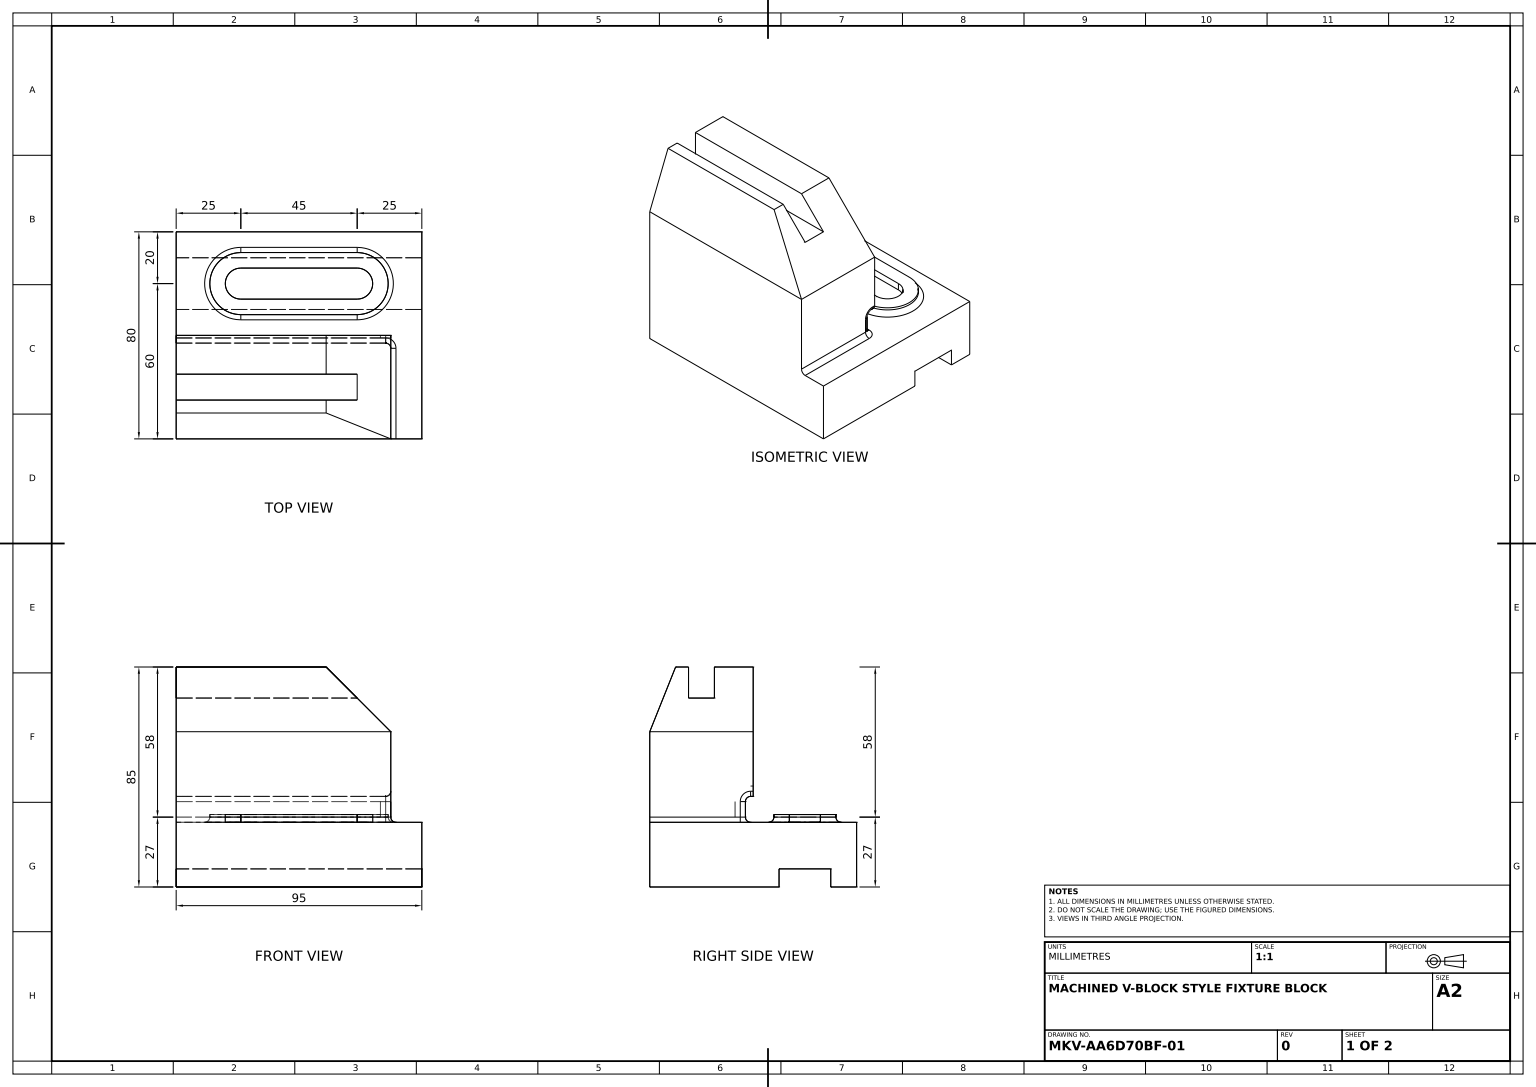
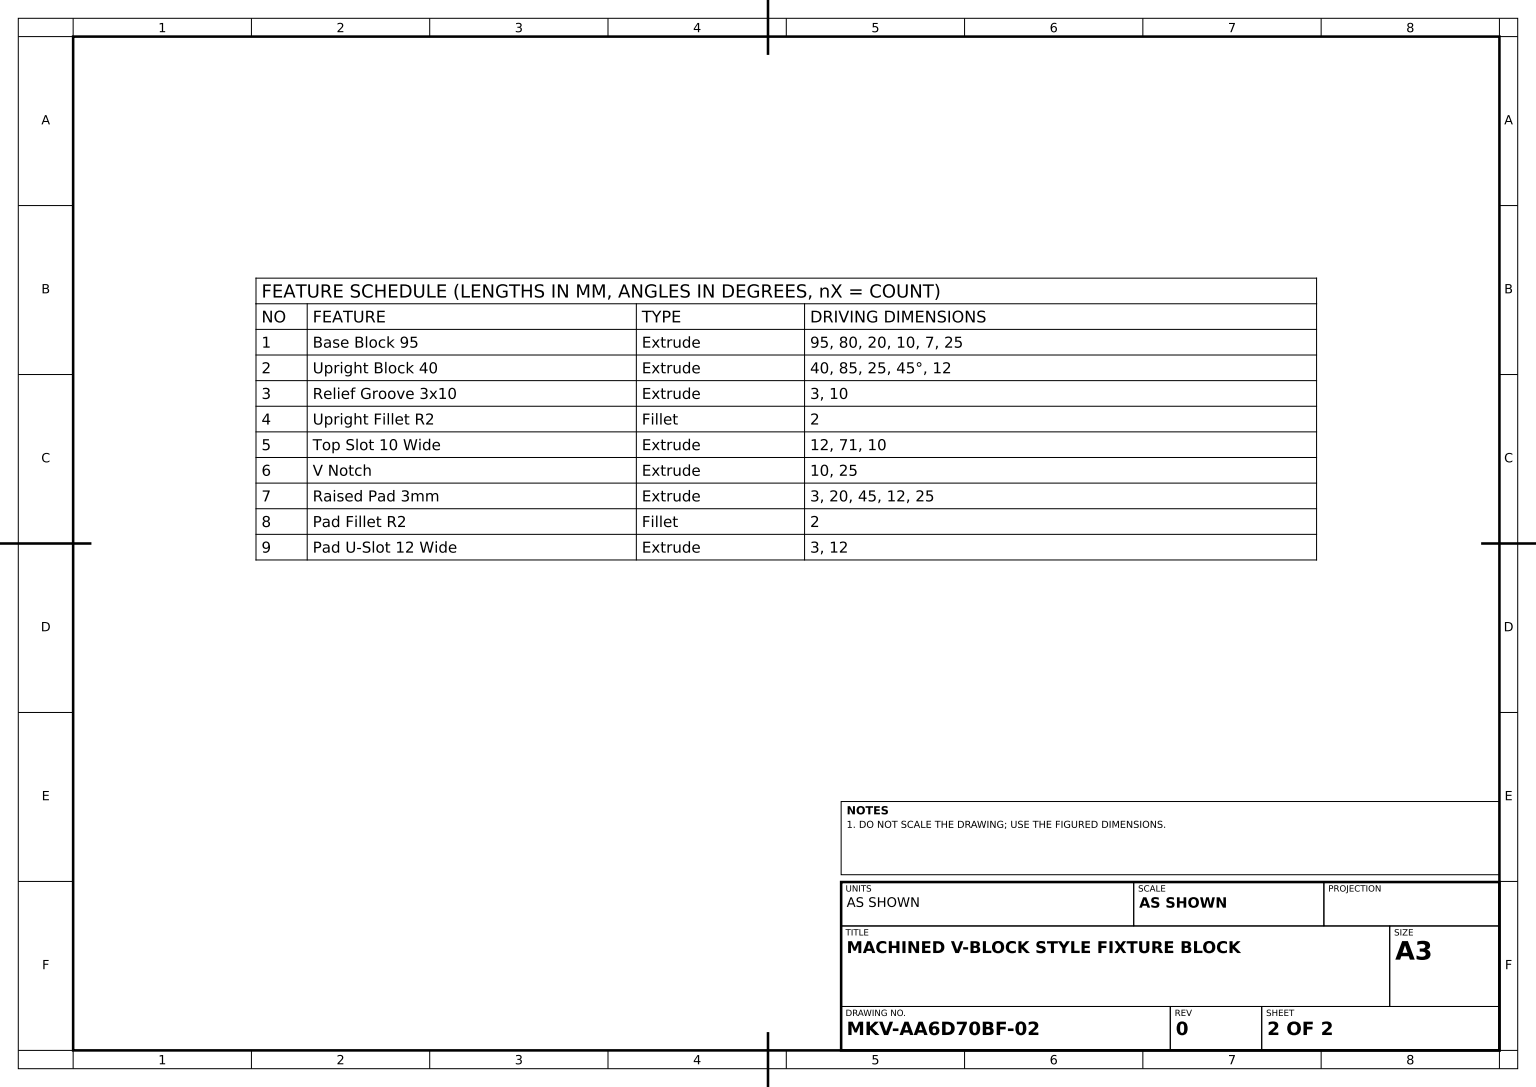
ISO-10303-21;
HEADER;
FILE_DESCRIPTION((''),'2;1');
FILE_NAME('','',(''),(''),'','','');
FILE_SCHEMA(('AUTOMOTIVE_DESIGN'));
ENDSEC;
DATA;
#1=APPLICATION_CONTEXT('');
#2=PRODUCT_CONTEXT('',#1,'mechanical');
#3=PRODUCT('','','',(#2));
#4=PRODUCT_DEFINITION_FORMATION('','',#3);
#5=PRODUCT_DEFINITION_CONTEXT('',#1,'design');
#6=PRODUCT_DEFINITION('','',#4,#5);
#7=PRODUCT_DEFINITION_SHAPE('','',#6);
#8=(LENGTH_UNIT()NAMED_UNIT(*)SI_UNIT(.MILLI.,.METRE.));
#9=(NAMED_UNIT(*)PLANE_ANGLE_UNIT()SI_UNIT($,.RADIAN.));
#10=(NAMED_UNIT(*)SI_UNIT($,.STERADIAN.)SOLID_ANGLE_UNIT());
#11=UNCERTAINTY_MEASURE_WITH_UNIT(LENGTH_MEASURE(1.E-05),#8,'distance_accuracy_value','');
#12=(GEOMETRIC_REPRESENTATION_CONTEXT(3)GLOBAL_UNCERTAINTY_ASSIGNED_CONTEXT((#11))GLOBAL_UNIT_ASSIGNED_CONTEXT((#8,#9,#10))REPRESENTATION_CONTEXT('',''));
#13=CARTESIAN_POINT('',(-22.5,27.,-48.));
#14=VERTEX_POINT('',#13);
#15=CARTESIAN_POINT('',(22.5,27.,-48.));
#16=VERTEX_POINT('',#15);
#17=DIRECTION('',(1.,0.,0.));
#18=VECTOR('',#17,1000.);
#19=LINE('',#15,#18);
#20=EDGE_CURVE('',#14,#16,#19,.T.);
#21=ORIENTED_EDGE('',*,*,#20,.F.);
#22=CARTESIAN_POINT('',(-22.5,25.,-46.));
#23=VERTEX_POINT('',#22);
#24=CARTESIAN_POINT('',(-22.5,27.,-46.));
#25=DIRECTION('',(-1.,0.,0.));
#26=DIRECTION('',(0.,0.,1.));
#27=AXIS2_PLACEMENT_3D('',#24,#25,#26);
#28=CIRCLE('',#27,2.);
#29=EDGE_CURVE('',#14,#23,#28,.T.);
#30=ORIENTED_EDGE('',*,*,#29,.T.);
#31=CARTESIAN_POINT('',(22.5,25.,-46.));
#32=VERTEX_POINT('',#31);
#33=VECTOR('',#25,1000.);
#34=LINE('',#22,#33);
#35=EDGE_CURVE('',#32,#23,#34,.T.);
#36=ORIENTED_EDGE('',*,*,#35,.F.);
#37=CARTESIAN_POINT('',(22.5,27.,-46.));
#38=AXIS2_PLACEMENT_3D('',#37,#25,#26);
#39=CIRCLE('',#38,2.);
#40=EDGE_CURVE('',#16,#32,#39,.T.);
#41=ORIENTED_EDGE('',*,*,#40,.F.);
#42=EDGE_LOOP('',(#21,#30,#36,#41));
#43=FACE_OUTER_BOUND('',#42,.T.);
#44=CYLINDRICAL_SURFACE('',#27,2.);
#45=ADVANCED_FACE('',(#43),#44,.F.);
#46=CARTESIAN_POINT('',(33.5,33.,-37.));
#47=VERTEX_POINT('',#46);
#48=CARTESIAN_POINT('',(33.5,35.,-39.));
#49=VERTEX_POINT('',#48);
#50=CARTESIAN_POINT('',(33.5,33.,-39.));
#51=DIRECTION('',(0.,0.,-1.));
#52=AXIS2_PLACEMENT_3D('',#50,#25,#51);
#53=CIRCLE('',#52,2.);
#54=EDGE_CURVE('',#47,#49,#53,.T.);
#55=ORIENTED_EDGE('',*,*,#54,.T.);
#56=CARTESIAN_POINT('',(35.5,37.,-39.));
#57=VERTEX_POINT('',#56);
#58=CARTESIAN_POINT('',(33.5,37.,-39.));
#59=AXIS2_PLACEMENT_3D('',#58,#51,#17);
#60=CIRCLE('',#59,2.);
#61=EDGE_CURVE('',#57,#49,#60,.T.);
#62=ORIENTED_EDGE('',*,*,#61,.F.);
#63=CARTESIAN_POINT('',(35.5,33.,-35.));
#64=VERTEX_POINT('',#63);
#65=CARTESIAN_POINT('',(35.5,33.,-39.));
#66=AXIS2_PLACEMENT_3D('',#65,#17,#51);
#67=CIRCLE('',#66,4.);
#68=EDGE_CURVE('',#57,#64,#67,.T.);
#69=ORIENTED_EDGE('',*,*,#68,.T.);
#70=CARTESIAN_POINT('',(33.5,33.,-35.));
#71=DIRECTION('',(0.,1.,0.));
#72=AXIS2_PLACEMENT_3D('',#70,#71,#26);
#73=CIRCLE('',#72,2.);
#74=EDGE_CURVE('',#64,#47,#73,.T.);
#75=ORIENTED_EDGE('',*,*,#74,.T.);
#76=EDGE_LOOP('',(#55,#62,#69,#75));
#77=FACE_OUTER_BOUND('',#76,.T.);
#78=AXIS2_PLACEMENT_3D('',#50,#17,#51);
#79=TOROIDAL_SURFACE('',#78,4.,2.);
#80=ADVANCED_FACE('',(#77),#79,.T.);
#81=CARTESIAN_POINT('',(33.5,27.,-37.));
#82=VERTEX_POINT('',#81);
#83=CARTESIAN_POINT('',(33.5,25.,-37.));
#84=DIRECTION('',(0.,-1.,0.));
#85=VECTOR('',#84,1000.);
#86=LINE('',#83,#85);
#87=EDGE_CURVE('',#47,#82,#86,.T.);
#88=ORIENTED_EDGE('',*,*,#87,.F.);
#89=ORIENTED_EDGE('',*,*,#74,.F.);
#90=CARTESIAN_POINT('',(35.5,27.,-35.));
#91=VERTEX_POINT('',#90);
#92=CARTESIAN_POINT('',(35.5,35.,-35.));
#93=VECTOR('',#71,1000.);
#94=LINE('',#92,#93);
#95=EDGE_CURVE('',#91,#64,#94,.T.);
#96=ORIENTED_EDGE('',*,*,#95,.F.);
#97=CARTESIAN_POINT('',(33.5,27.,-35.));
#98=AXIS2_PLACEMENT_3D('',#97,#71,#51);
#99=CIRCLE('',#98,2.);
#100=EDGE_CURVE('',#91,#82,#99,.T.);
#101=ORIENTED_EDGE('',*,*,#100,.T.);
#102=EDGE_LOOP('',(#88,#89,#96,#101));
#103=FACE_OUTER_BOUND('',#102,.T.);
#104=CARTESIAN_POINT('',(33.5,35.,-35.));
#105=AXIS2_PLACEMENT_3D('',#104,#71,#26);
#106=CYLINDRICAL_SURFACE('',#105,2.);
#107=ADVANCED_FACE('',(#103),#106,.T.);
#108=CARTESIAN_POINT('',(35.5,60.,0.));
#109=VERTEX_POINT('',#108);
#110=CARTESIAN_POINT('',(-47.5,60.,0.));
#111=VERTEX_POINT('',#110);
#112=CARTESIAN_POINT('',(47.5,60.,0.));
#113=LINE('',#112,#33);
#114=EDGE_CURVE('',#109,#111,#113,.T.);
#115=ORIENTED_EDGE('',*,*,#114,.T.);
#116=CARTESIAN_POINT('',(-47.5,0.,0.));
#117=VERTEX_POINT('',#116);
#118=CARTESIAN_POINT('',(-47.5,25.,0.));
#119=LINE('',#118,#85);
#120=EDGE_CURVE('',#111,#117,#119,.T.);
#121=ORIENTED_EDGE('',*,*,#120,.T.);
#122=CARTESIAN_POINT('',(47.5,0.,0.));
#123=VERTEX_POINT('',#122);
#124=LINE('',#122,#33);
#125=EDGE_CURVE('',#123,#117,#124,.T.);
#126=ORIENTED_EDGE('',*,*,#125,.F.);
#127=CARTESIAN_POINT('',(47.5,25.,0.));
#128=VERTEX_POINT('',#127);
#129=LINE('',#127,#85);
#130=EDGE_CURVE('',#128,#123,#129,.T.);
#131=ORIENTED_EDGE('',*,*,#130,.F.);
#132=CARTESIAN_POINT('',(37.5,25.,0.));
#133=VERTEX_POINT('',#132);
#134=LINE('',#127,#33);
#135=EDGE_CURVE('',#128,#133,#134,.T.);
#136=ORIENTED_EDGE('',*,*,#135,.T.);
#137=CARTESIAN_POINT('',(35.5,27.,0.));
#138=VERTEX_POINT('',#137);
#139=CARTESIAN_POINT('',(37.5,27.,0.));
#140=AXIS2_PLACEMENT_3D('',#139,#51,#71);
#141=CIRCLE('',#140,2.);
#142=EDGE_CURVE('',#133,#138,#141,.T.);
#143=ORIENTED_EDGE('',*,*,#142,.T.);
#144=LINE('',#108,#93);
#145=EDGE_CURVE('',#138,#109,#144,.T.);
#146=ORIENTED_EDGE('',*,*,#145,.T.);
#147=EDGE_LOOP('',(#115,#121,#126,#131,#136,#143,#146));
#148=FACE_OUTER_BOUND('',#147,.T.);
#149=AXIS2_PLACEMENT_3D('',#127,#51,#71);
#150=PLANE('',#149);
#151=ADVANCED_FACE('',(#148),#150,.F.);
#152=CARTESIAN_POINT('',(10.5,85.,-40.));
#153=VERTEX_POINT('',#152);
#154=CARTESIAN_POINT('',(10.5,85.,-25.));
#155=VERTEX_POINT('',#154);
#156=VECTOR('',#26,1000.);
#157=LINE('',#152,#156);
#158=EDGE_CURVE('',#153,#155,#157,.T.);
#159=ORIENTED_EDGE('',*,*,#158,.F.);
#160=CARTESIAN_POINT('',(-47.5,85.,-40.));
#161=VERTEX_POINT('',#160);
#162=LINE('',#160,#33);
#163=EDGE_CURVE('',#153,#161,#162,.T.);
#164=ORIENTED_EDGE('',*,*,#163,.T.);
#165=CARTESIAN_POINT('',(-47.5,85.,-25.));
#166=VERTEX_POINT('',#165);
#167=LINE('',#160,#156);
#168=EDGE_CURVE('',#161,#166,#167,.T.);
#169=ORIENTED_EDGE('',*,*,#168,.T.);
#170=LINE('',#165,#18);
#171=EDGE_CURVE('',#166,#155,#170,.T.);
#172=ORIENTED_EDGE('',*,*,#171,.T.);
#173=EDGE_LOOP('',(#159,#164,#169,#172));
#174=FACE_OUTER_BOUND('',#173,.T.);
#175=AXIS2_PLACEMENT_3D('',#160,#71,#26);
#176=PLANE('',#175);
#177=ADVANCED_FACE('',(#174),#176,.T.);
#178=CARTESIAN_POINT('',(-22.5,25.,-66.));
#179=VERTEX_POINT('',#178);
#180=CARTESIAN_POINT('',(-22.5,25.,-54.));
#181=VERTEX_POINT('',#180);
#182=CARTESIAN_POINT('',(-22.5,25.,-60.));
#183=AXIS2_PLACEMENT_3D('',#182,#71,#26);
#184=CIRCLE('',#183,6.);
#185=EDGE_CURVE('',#179,#181,#184,.T.);
#186=ORIENTED_EDGE('',*,*,#185,.T.);
#187=CARTESIAN_POINT('',(22.5,25.,-54.));
#188=VERTEX_POINT('',#187);
#189=LINE('',#180,#18);
#190=EDGE_CURVE('',#181,#188,#189,.T.);
#191=ORIENTED_EDGE('',*,*,#190,.T.);
#192=CARTESIAN_POINT('',(22.5,25.,-66.));
#193=VERTEX_POINT('',#192);
#194=CARTESIAN_POINT('',(22.5,25.,-60.));
#195=AXIS2_PLACEMENT_3D('',#194,#71,#26);
#196=CIRCLE('',#195,6.);
#197=EDGE_CURVE('',#188,#193,#196,.T.);
#198=ORIENTED_EDGE('',*,*,#197,.T.);
#199=LINE('',#178,#33);
#200=EDGE_CURVE('',#193,#179,#199,.T.);
#201=ORIENTED_EDGE('',*,*,#200,.T.);
#202=EDGE_LOOP('',(#186,#191,#198,#201));
#203=FACE_OUTER_BOUND('',#202,.T.);
#204=PLANE('',#183);
#205=ADVANCED_FACE('',(#203),#204,.T.);
#206=ORIENTED_EDGE('',*,*,#197,.F.);
#207=CARTESIAN_POINT('',(22.5,28.,-54.));
#208=VERTEX_POINT('',#207);
#209=LINE('',#187,#93);
#210=EDGE_CURVE('',#188,#208,#209,.T.);
#211=ORIENTED_EDGE('',*,*,#210,.T.);
#212=CARTESIAN_POINT('',(22.5,28.,-66.));
#213=VERTEX_POINT('',#212);
#214=CARTESIAN_POINT('',(22.5,28.,-60.));
#215=AXIS2_PLACEMENT_3D('',#214,#71,#26);
#216=CIRCLE('',#215,6.);
#217=EDGE_CURVE('',#208,#213,#216,.T.);
#218=ORIENTED_EDGE('',*,*,#217,.T.);
#219=LINE('',#192,#93);
#220=EDGE_CURVE('',#193,#213,#219,.T.);
#221=ORIENTED_EDGE('',*,*,#220,.F.);
#222=EDGE_LOOP('',(#206,#211,#218,#221));
#223=FACE_OUTER_BOUND('',#222,.T.);
#224=CYLINDRICAL_SURFACE('',#195,6.);
#225=ADVANCED_FACE('',(#223),#224,.F.);
#226=CARTESIAN_POINT('',(-47.5,73.,-15.));
#227=VERTEX_POINT('',#226);
#228=CARTESIAN_POINT('',(-47.5,73.,-25.));
#229=VERTEX_POINT('',#228);
#230=VECTOR('',#51,1000.);
#231=LINE('',#226,#230);
#232=EDGE_CURVE('',#227,#229,#231,.T.);
#233=ORIENTED_EDGE('',*,*,#232,.T.);
#234=LINE('',#228,#93);
#235=EDGE_CURVE('',#229,#166,#234,.T.);
#236=ORIENTED_EDGE('',*,*,#235,.T.);
#237=ORIENTED_EDGE('',*,*,#168,.F.);
#238=CARTESIAN_POINT('',(-47.5,35.,-40.));
#239=VERTEX_POINT('',#238);
#240=CARTESIAN_POINT('',(-47.5,25.,-40.));
#241=LINE('',#240,#85);
#242=EDGE_CURVE('',#161,#239,#241,.T.);
#243=ORIENTED_EDGE('',*,*,#242,.T.);
#244=CARTESIAN_POINT('',(-47.5,35.,-39.));
#245=VERTEX_POINT('',#244);
#246=LINE('',#238,#156);
#247=EDGE_CURVE('',#239,#245,#246,.T.);
#248=ORIENTED_EDGE('',*,*,#247,.T.);
#249=CARTESIAN_POINT('',(-47.5,33.,-37.));
#250=VERTEX_POINT('',#249);
#251=CARTESIAN_POINT('',(-47.5,33.,-39.));
#252=AXIS2_PLACEMENT_3D('',#251,#17,#51);
#253=CIRCLE('',#252,2.);
#254=EDGE_CURVE('',#245,#250,#253,.T.);
#255=ORIENTED_EDGE('',*,*,#254,.T.);
#256=CARTESIAN_POINT('',(-47.5,27.,-37.));
#257=VERTEX_POINT('',#256);
#258=CARTESIAN_POINT('',(-47.5,35.,-37.));
#259=LINE('',#258,#85);
#260=EDGE_CURVE('',#250,#257,#259,.T.);
#261=ORIENTED_EDGE('',*,*,#260,.T.);
#262=CARTESIAN_POINT('',(-47.5,25.,-39.));
#263=VERTEX_POINT('',#262);
#264=CARTESIAN_POINT('',(-47.5,27.,-39.));
#265=AXIS2_PLACEMENT_3D('',#264,#17,#51);
#266=CIRCLE('',#265,2.);
#267=EDGE_CURVE('',#257,#263,#266,.T.);
#268=ORIENTED_EDGE('',*,*,#267,.T.);
#269=CARTESIAN_POINT('',(-47.5,25.,-80.));
#270=VERTEX_POINT('',#269);
#271=LINE('',#269,#156);
#272=EDGE_CURVE('',#270,#263,#271,.T.);
#273=ORIENTED_EDGE('',*,*,#272,.F.);
#274=CARTESIAN_POINT('',(-47.5,0.,-80.));
#275=VERTEX_POINT('',#274);
#276=LINE('',#274,#93);
#277=EDGE_CURVE('',#275,#270,#276,.T.);
#278=ORIENTED_EDGE('',*,*,#277,.F.);
#279=CARTESIAN_POINT('',(-47.5,0.,-70.));
#280=VERTEX_POINT('',#279);
#281=LINE('',#279,#230);
#282=EDGE_CURVE('',#280,#275,#281,.T.);
#283=ORIENTED_EDGE('',*,*,#282,.F.);
#284=CARTESIAN_POINT('',(-47.5,7.,-70.));
#285=VERTEX_POINT('',#284);
#286=LINE('',#284,#85);
#287=EDGE_CURVE('',#285,#280,#286,.T.);
#288=ORIENTED_EDGE('',*,*,#287,.F.);
#289=CARTESIAN_POINT('',(-47.5,7.,-50.));
#290=VERTEX_POINT('',#289);
#291=LINE('',#289,#230);
#292=EDGE_CURVE('',#290,#285,#291,.T.);
#293=ORIENTED_EDGE('',*,*,#292,.F.);
#294=CARTESIAN_POINT('',(-47.5,0.,-50.));
#295=VERTEX_POINT('',#294);
#296=LINE('',#294,#93);
#297=EDGE_CURVE('',#295,#290,#296,.T.);
#298=ORIENTED_EDGE('',*,*,#297,.F.);
#299=LINE('',#116,#230);
#300=EDGE_CURVE('',#117,#295,#299,.T.);
#301=ORIENTED_EDGE('',*,*,#300,.F.);
#302=ORIENTED_EDGE('',*,*,#120,.F.);
#303=CARTESIAN_POINT('',(-47.5,85.,-10.));
#304=VERTEX_POINT('',#303);
#305=DIRECTION('',(0.,-0.928476691,0.371390676));
#306=VECTOR('',#305,1000.);
#307=LINE('',#303,#306);
#308=EDGE_CURVE('',#304,#111,#307,.T.);
#309=ORIENTED_EDGE('',*,*,#308,.F.);
#310=CARTESIAN_POINT('',(-47.5,85.,-15.));
#311=VERTEX_POINT('',#310);
#312=EDGE_CURVE('',#311,#304,#167,.T.);
#313=ORIENTED_EDGE('',*,*,#312,.F.);
#314=LINE('',#226,#93);
#315=EDGE_CURVE('',#227,#311,#314,.T.);
#316=ORIENTED_EDGE('',*,*,#315,.F.);
#317=EDGE_LOOP('',(#233,#236,#237,#243,#248,#255,#261,#268,#273,#278,#283,#288,#293,#298,#301,#302,#309,#313,#316));
#318=FACE_OUTER_BOUND('',#317,.T.);
#319=AXIS2_PLACEMENT_3D('',#116,#17,#51);
#320=PLANE('',#319);
#321=ADVANCED_FACE('',(#318),#320,.F.);
#322=CARTESIAN_POINT('',(22.5,28.,-72.));
#323=VERTEX_POINT('',#322);
#324=CARTESIAN_POINT('',(22.5,27.,-72.));
#325=VERTEX_POINT('',#324);
#326=LINE('',#322,#85);
#327=EDGE_CURVE('',#323,#325,#326,.T.);
#328=ORIENTED_EDGE('',*,*,#327,.F.);
#329=CARTESIAN_POINT('',(22.5,28.,-48.));
#330=VERTEX_POINT('',#329);
#331=CIRCLE('',#215,12.);
#332=EDGE_CURVE('',#330,#323,#331,.T.);
#333=ORIENTED_EDGE('',*,*,#332,.F.);
#334=LINE('',#329,#85);
#335=EDGE_CURVE('',#330,#16,#334,.T.);
#336=ORIENTED_EDGE('',*,*,#335,.T.);
#337=CARTESIAN_POINT('',(22.5,27.,-60.));
#338=AXIS2_PLACEMENT_3D('',#337,#71,#51);
#339=CIRCLE('',#338,12.);
#340=EDGE_CURVE('',#16,#325,#339,.T.);
#341=ORIENTED_EDGE('',*,*,#340,.T.);
#342=EDGE_LOOP('',(#328,#333,#336,#341));
#343=FACE_OUTER_BOUND('',#342,.T.);
#344=AXIS2_PLACEMENT_3D('',#214,#84,#51);
#345=CYLINDRICAL_SURFACE('',#344,12.);
#346=ADVANCED_FACE('',(#343),#345,.T.);
#347=CARTESIAN_POINT('',(47.5,0.,-80.));
#348=VERTEX_POINT('',#347);
#349=LINE('',#347,#33);
#350=EDGE_CURVE('',#348,#275,#349,.T.);
#351=ORIENTED_EDGE('',*,*,#350,.F.);
#352=CARTESIAN_POINT('',(47.5,0.,-70.));
#353=VERTEX_POINT('',#352);
#354=LINE('',#352,#230);
#355=EDGE_CURVE('',#353,#348,#354,.T.);
#356=ORIENTED_EDGE('',*,*,#355,.F.);
#357=LINE('',#352,#33);
#358=EDGE_CURVE('',#353,#280,#357,.T.);
#359=ORIENTED_EDGE('',*,*,#358,.T.);
#360=ORIENTED_EDGE('',*,*,#282,.T.);
#361=EDGE_LOOP('',(#351,#356,#359,#360));
#362=FACE_OUTER_BOUND('',#361,.T.);
#363=AXIS2_PLACEMENT_3D('',#352,#71,#26);
#364=PLANE('',#363);
#365=ADVANCED_FACE('',(#362),#364,.F.);
#366=ORIENTED_EDGE('',*,*,#355,.T.);
#367=CARTESIAN_POINT('',(47.5,25.,-80.));
#368=VERTEX_POINT('',#367);
#369=LINE('',#347,#93);
#370=EDGE_CURVE('',#348,#368,#369,.T.);
#371=ORIENTED_EDGE('',*,*,#370,.T.);
#372=LINE('',#367,#156);
#373=EDGE_CURVE('',#368,#128,#372,.T.);
#374=ORIENTED_EDGE('',*,*,#373,.T.);
#375=ORIENTED_EDGE('',*,*,#130,.T.);
#376=CARTESIAN_POINT('',(47.5,0.,-50.));
#377=VERTEX_POINT('',#376);
#378=LINE('',#122,#230);
#379=EDGE_CURVE('',#123,#377,#378,.T.);
#380=ORIENTED_EDGE('',*,*,#379,.T.);
#381=CARTESIAN_POINT('',(47.5,7.,-50.));
#382=VERTEX_POINT('',#381);
#383=LINE('',#376,#93);
#384=EDGE_CURVE('',#377,#382,#383,.T.);
#385=ORIENTED_EDGE('',*,*,#384,.T.);
#386=CARTESIAN_POINT('',(47.5,7.,-70.));
#387=VERTEX_POINT('',#386);
#388=LINE('',#381,#230);
#389=EDGE_CURVE('',#382,#387,#388,.T.);
#390=ORIENTED_EDGE('',*,*,#389,.T.);
#391=LINE('',#386,#85);
#392=EDGE_CURVE('',#387,#353,#391,.T.);
#393=ORIENTED_EDGE('',*,*,#392,.T.);
#394=EDGE_LOOP('',(#366,#371,#374,#375,#380,#385,#390,#393));
#395=FACE_OUTER_BOUND('',#394,.T.);
#396=AXIS2_PLACEMENT_3D('',#122,#17,#51);
#397=PLANE('',#396);
#398=ADVANCED_FACE('',(#395),#397,.T.);
#399=ORIENTED_EDGE('',*,*,#190,.F.);
#400=CARTESIAN_POINT('',(-22.5,28.,-54.));
#401=VERTEX_POINT('',#400);
#402=LINE('',#180,#93);
#403=EDGE_CURVE('',#181,#401,#402,.T.);
#404=ORIENTED_EDGE('',*,*,#403,.T.);
#405=LINE('',#400,#18);
#406=EDGE_CURVE('',#401,#208,#405,.T.);
#407=ORIENTED_EDGE('',*,*,#406,.T.);
#408=ORIENTED_EDGE('',*,*,#210,.F.);
#409=EDGE_LOOP('',(#399,#404,#407,#408));
#410=FACE_OUTER_BOUND('',#409,.T.);
#411=AXIS2_PLACEMENT_3D('',#180,#26,#84);
#412=PLANE('',#411);
#413=ADVANCED_FACE('',(#410),#412,.F.);
#414=ORIENTED_EDGE('',*,*,#254,.F.);
#415=LINE('',#244,#33);
#416=EDGE_CURVE('',#49,#245,#415,.T.);
#417=ORIENTED_EDGE('',*,*,#416,.F.);
#418=ORIENTED_EDGE('',*,*,#54,.F.);
#419=CARTESIAN_POINT('',(35.5,33.,-37.));
#420=LINE('',#419,#18);
#421=EDGE_CURVE('',#250,#47,#420,.T.);
#422=ORIENTED_EDGE('',*,*,#421,.F.);
#423=EDGE_LOOP('',(#414,#417,#418,#422));
#424=FACE_OUTER_BOUND('',#423,.T.);
#425=AXIS2_PLACEMENT_3D('',#251,#25,#26);
#426=CYLINDRICAL_SURFACE('',#425,2.);
#427=ADVANCED_FACE('',(#424),#426,.F.);
#428=CARTESIAN_POINT('',(10.5,85.,-10.));
#429=VERTEX_POINT('',#428);
#430=LINE('',#303,#33);
#431=EDGE_CURVE('',#429,#304,#430,.T.);
#432=ORIENTED_EDGE('',*,*,#431,.T.);
#433=ORIENTED_EDGE('',*,*,#308,.T.);
#434=ORIENTED_EDGE('',*,*,#114,.F.);
#435=CARTESIAN_POINT('',(4.944444,90.555556,-12.222222));
#436=DIRECTION('',(-0.680413817,0.680413817,-0.272165527));
#437=VECTOR('',#436,1000.);
#438=LINE('',#435,#437);
#439=EDGE_CURVE('',#109,#429,#438,.T.);
#440=ORIENTED_EDGE('',*,*,#439,.T.);
#441=EDGE_LOOP('',(#432,#433,#434,#440));
#442=FACE_OUTER_BOUND('',#441,.T.);
#443=CARTESIAN_POINT('',(47.5,85.,-10.));
#444=DIRECTION('',(0.,-0.371390676,-0.928476691));
#445=DIRECTION('',(0.,0.928476691,-0.371390676));
#446=AXIS2_PLACEMENT_3D('',#443,#444,#445);
#447=PLANE('',#446);
#448=ADVANCED_FACE('',(#442),#447,.F.);
#449=LINE('',#256,#33);
#450=EDGE_CURVE('',#82,#257,#449,.T.);
#451=ORIENTED_EDGE('',*,*,#450,.T.);
#452=ORIENTED_EDGE('',*,*,#260,.F.);
#453=ORIENTED_EDGE('',*,*,#421,.T.);
#454=ORIENTED_EDGE('',*,*,#87,.T.);
#455=EDGE_LOOP('',(#451,#452,#453,#454));
#456=FACE_OUTER_BOUND('',#455,.T.);
#457=AXIS2_PLACEMENT_3D('',#258,#26,#17);
#458=PLANE('',#457);
#459=ADVANCED_FACE('',(#456),#458,.F.);
#460=LINE('',#386,#33);
#461=EDGE_CURVE('',#387,#285,#460,.T.);
#462=ORIENTED_EDGE('',*,*,#461,.T.);
#463=ORIENTED_EDGE('',*,*,#287,.T.);
#464=ORIENTED_EDGE('',*,*,#358,.F.);
#465=ORIENTED_EDGE('',*,*,#392,.F.);
#466=EDGE_LOOP('',(#462,#463,#464,#465));
#467=FACE_OUTER_BOUND('',#466,.T.);
#468=AXIS2_PLACEMENT_3D('',#386,#51,#25);
#469=PLANE('',#468);
#470=ADVANCED_FACE('',(#467),#469,.F.);
#471=CARTESIAN_POINT('',(-22.5,28.,-48.));
#472=VERTEX_POINT('',#471);
#473=LINE('',#471,#85);
#474=EDGE_CURVE('',#472,#14,#473,.T.);
#475=ORIENTED_EDGE('',*,*,#474,.F.);
#476=CARTESIAN_POINT('',(-22.5,28.,-72.));
#477=VERTEX_POINT('',#476);
#478=CARTESIAN_POINT('',(-22.5,28.,-60.));
#479=AXIS2_PLACEMENT_3D('',#478,#71,#26);
#480=CIRCLE('',#479,12.);
#481=EDGE_CURVE('',#477,#472,#480,.T.);
#482=ORIENTED_EDGE('',*,*,#481,.F.);
#483=CARTESIAN_POINT('',(-22.5,27.,-72.));
#484=VERTEX_POINT('',#483);
#485=LINE('',#476,#85);
#486=EDGE_CURVE('',#477,#484,#485,.T.);
#487=ORIENTED_EDGE('',*,*,#486,.T.);
#488=CARTESIAN_POINT('',(-22.5,27.,-60.));
#489=AXIS2_PLACEMENT_3D('',#488,#71,#51);
#490=CIRCLE('',#489,12.);
#491=EDGE_CURVE('',#484,#14,#490,.T.);
#492=ORIENTED_EDGE('',*,*,#491,.T.);
#493=EDGE_LOOP('',(#475,#482,#487,#492));
#494=FACE_OUTER_BOUND('',#493,.T.);
#495=AXIS2_PLACEMENT_3D('',#478,#84,#51);
#496=CYLINDRICAL_SURFACE('',#495,12.);
#497=ADVANCED_FACE('',(#494),#496,.T.);
#498=CARTESIAN_POINT('',(10.5,85.,-15.));
#499=VERTEX_POINT('',#498);
#500=LINE('',#310,#18);
#501=EDGE_CURVE('',#311,#499,#500,.T.);
#502=ORIENTED_EDGE('',*,*,#501,.F.);
#503=ORIENTED_EDGE('',*,*,#312,.T.);
#504=ORIENTED_EDGE('',*,*,#431,.F.);
#505=EDGE_CURVE('',#499,#429,#157,.T.);
#506=ORIENTED_EDGE('',*,*,#505,.F.);
#507=EDGE_LOOP('',(#502,#503,#504,#506));
#508=FACE_OUTER_BOUND('',#507,.T.);
#509=ADVANCED_FACE('',(#508),#176,.T.);
#510=CARTESIAN_POINT('',(22.5,25.,-74.));
#511=VERTEX_POINT('',#510);
#512=AXIS2_PLACEMENT_3D('',#194,#84,#51);
#513=CIRCLE('',#512,14.);
#514=EDGE_CURVE('',#511,#32,#513,.T.);
#515=ORIENTED_EDGE('',*,*,#514,.F.);
#516=CARTESIAN_POINT('',(22.5,27.,-74.));
#517=AXIS2_PLACEMENT_3D('',#516,#25,#26);
#518=CIRCLE('',#517,2.);
#519=EDGE_CURVE('',#511,#325,#518,.T.);
#520=ORIENTED_EDGE('',*,*,#519,.T.);
#521=ORIENTED_EDGE('',*,*,#340,.F.);
#522=ORIENTED_EDGE('',*,*,#40,.T.);
#523=EDGE_LOOP('',(#515,#520,#521,#522));
#524=FACE_OUTER_BOUND('',#523,.T.);
#525=AXIS2_PLACEMENT_3D('',#337,#84,#51);
#526=TOROIDAL_SURFACE('',#525,14.,2.);
#527=ADVANCED_FACE('',(#524),#526,.F.);
#528=ORIENTED_EDGE('',*,*,#142,.F.);
#529=CARTESIAN_POINT('',(37.5,25.,-35.));
#530=VERTEX_POINT('',#529);
#531=CARTESIAN_POINT('',(37.5,25.,-80.));
#532=LINE('',#531,#156);
#533=EDGE_CURVE('',#530,#133,#532,.T.);
#534=ORIENTED_EDGE('',*,*,#533,.F.);
#535=CARTESIAN_POINT('',(37.5,27.,-35.));
#536=AXIS2_PLACEMENT_3D('',#535,#26,#17);
#537=CIRCLE('',#536,2.);
#538=EDGE_CURVE('',#91,#530,#537,.T.);
#539=ORIENTED_EDGE('',*,*,#538,.F.);
#540=CARTESIAN_POINT('',(35.5,27.,-40.));
#541=LINE('',#540,#230);
#542=EDGE_CURVE('',#138,#91,#541,.T.);
#543=ORIENTED_EDGE('',*,*,#542,.F.);
#544=EDGE_LOOP('',(#528,#534,#539,#543));
#545=FACE_OUTER_BOUND('',#544,.T.);
#546=CARTESIAN_POINT('',(37.5,27.,-80.));
#547=AXIS2_PLACEMENT_3D('',#546,#26,#84);
#548=CYLINDRICAL_SURFACE('',#547,2.);
#549=ADVANCED_FACE('',(#545),#548,.F.);
#550=ORIENTED_EDGE('',*,*,#163,.F.);
#551=CARTESIAN_POINT('',(35.5,60.,-40.));
#552=VERTEX_POINT('',#551);
#553=DIRECTION('',(-0.707106781,0.707106781,0.));
#554=VECTOR('',#553,1000.);
#555=LINE('',#152,#554);
#556=EDGE_CURVE('',#552,#153,#555,.T.);
#557=ORIENTED_EDGE('',*,*,#556,.F.);
#558=CARTESIAN_POINT('',(35.5,37.,-40.));
#559=VERTEX_POINT('',#558);
#560=LINE('',#551,#93);
#561=EDGE_CURVE('',#559,#552,#560,.T.);
#562=ORIENTED_EDGE('',*,*,#561,.F.);
#563=CARTESIAN_POINT('',(33.5,35.,-40.));
#564=VERTEX_POINT('',#563);
#565=CARTESIAN_POINT('',(33.5,37.,-40.));
#566=AXIS2_PLACEMENT_3D('',#565,#51,#25);
#567=CIRCLE('',#566,2.);
#568=EDGE_CURVE('',#559,#564,#567,.T.);
#569=ORIENTED_EDGE('',*,*,#568,.T.);
#570=LINE('',#238,#18);
#571=EDGE_CURVE('',#239,#564,#570,.T.);
#572=ORIENTED_EDGE('',*,*,#571,.F.);
#573=ORIENTED_EDGE('',*,*,#242,.F.);
#574=EDGE_LOOP('',(#550,#557,#562,#569,#572,#573));
#575=FACE_OUTER_BOUND('',#574,.T.);
#576=CARTESIAN_POINT('',(0.,0.,-40.));
#577=AXIS2_PLACEMENT_3D('',#576,#51,#25);
#578=PLANE('',#577);
#579=ADVANCED_FACE('',(#575),#578,.T.);
#580=LINE('',#558,#230);
#581=EDGE_CURVE('',#57,#559,#580,.T.);
#582=ORIENTED_EDGE('',*,*,#581,.T.);
#583=ORIENTED_EDGE('',*,*,#561,.T.);
#584=LINE('',#551,#156);
#585=EDGE_CURVE('',#552,#109,#584,.T.);
#586=ORIENTED_EDGE('',*,*,#585,.T.);
#587=ORIENTED_EDGE('',*,*,#145,.F.);
#588=ORIENTED_EDGE('',*,*,#542,.T.);
#589=ORIENTED_EDGE('',*,*,#95,.T.);
#590=ORIENTED_EDGE('',*,*,#68,.F.);
#591=EDGE_LOOP('',(#582,#583,#586,#587,#588,#589,#590));
#592=FACE_OUTER_BOUND('',#591,.T.);
#593=AXIS2_PLACEMENT_3D('',#551,#17,#51);
#594=PLANE('',#593);
#595=ADVANCED_FACE('',(#592),#594,.T.);
#596=LINE('',#381,#33);
#597=EDGE_CURVE('',#382,#290,#596,.T.);
#598=ORIENTED_EDGE('',*,*,#597,.F.);
#599=ORIENTED_EDGE('',*,*,#384,.F.);
#600=LINE('',#376,#33);
#601=EDGE_CURVE('',#377,#295,#600,.T.);
#602=ORIENTED_EDGE('',*,*,#601,.T.);
#603=ORIENTED_EDGE('',*,*,#297,.T.);
#604=EDGE_LOOP('',(#598,#599,#602,#603));
#605=FACE_OUTER_BOUND('',#604,.T.);
#606=AXIS2_PLACEMENT_3D('',#376,#26,#17);
#607=PLANE('',#606);
#608=ADVANCED_FACE('',(#605),#607,.F.);
#609=LINE('',#471,#18);
#610=EDGE_CURVE('',#472,#330,#609,.T.);
#611=ORIENTED_EDGE('',*,*,#610,.F.);
#612=ORIENTED_EDGE('',*,*,#474,.T.);
#613=ORIENTED_EDGE('',*,*,#20,.T.);
#614=ORIENTED_EDGE('',*,*,#335,.F.);
#615=EDGE_LOOP('',(#611,#612,#613,#614));
#616=FACE_OUTER_BOUND('',#615,.T.);
#617=AXIS2_PLACEMENT_3D('',#471,#51,#25);
#618=PLANE('',#617);
#619=ADVANCED_FACE('',(#616),#618,.F.);
#620=ORIENTED_EDGE('',*,*,#350,.T.);
#621=ORIENTED_EDGE('',*,*,#277,.T.);
#622=LINE('',#367,#33);
#623=EDGE_CURVE('',#368,#270,#622,.T.);
#624=ORIENTED_EDGE('',*,*,#623,.F.);
#625=ORIENTED_EDGE('',*,*,#370,.F.);
#626=EDGE_LOOP('',(#620,#621,#624,#625));
#627=FACE_OUTER_BOUND('',#626,.T.);
#628=AXIS2_PLACEMENT_3D('',#347,#26,#17);
#629=PLANE('',#628);
#630=ADVANCED_FACE('',(#627),#629,.F.);
#631=LINE('',#483,#33);
#632=EDGE_CURVE('',#325,#484,#631,.T.);
#633=ORIENTED_EDGE('',*,*,#632,.F.);
#634=ORIENTED_EDGE('',*,*,#519,.F.);
#635=CARTESIAN_POINT('',(-22.5,25.,-74.));
#636=VERTEX_POINT('',#635);
#637=LINE('',#510,#18);
#638=EDGE_CURVE('',#636,#511,#637,.T.);
#639=ORIENTED_EDGE('',*,*,#638,.F.);
#640=CARTESIAN_POINT('',(-22.5,27.,-74.));
#641=AXIS2_PLACEMENT_3D('',#640,#25,#26);
#642=CIRCLE('',#641,2.);
#643=EDGE_CURVE('',#636,#484,#642,.T.);
#644=ORIENTED_EDGE('',*,*,#643,.T.);
#645=EDGE_LOOP('',(#633,#634,#639,#644));
#646=FACE_OUTER_BOUND('',#645,.T.);
#647=AXIS2_PLACEMENT_3D('',#640,#17,#51);
#648=CYLINDRICAL_SURFACE('',#647,2.);
#649=ADVANCED_FACE('',(#646),#648,.F.);
#650=ORIENTED_EDGE('',*,*,#217,.F.);
#651=ORIENTED_EDGE('',*,*,#406,.F.);
#652=CARTESIAN_POINT('',(-22.5,28.,-66.));
#653=VERTEX_POINT('',#652);
#654=CIRCLE('',#479,6.);
#655=EDGE_CURVE('',#653,#401,#654,.T.);
#656=ORIENTED_EDGE('',*,*,#655,.F.);
#657=LINE('',#652,#33);
#658=EDGE_CURVE('',#213,#653,#657,.T.);
#659=ORIENTED_EDGE('',*,*,#658,.F.);
#660=EDGE_LOOP('',(#650,#651,#656,#659));
#661=FACE_BOUND('',#660,.T.);
#662=ORIENTED_EDGE('',*,*,#610,.T.);
#663=ORIENTED_EDGE('',*,*,#332,.T.);
#664=LINE('',#476,#33);
#665=EDGE_CURVE('',#323,#477,#664,.T.);
#666=ORIENTED_EDGE('',*,*,#665,.T.);
#667=ORIENTED_EDGE('',*,*,#481,.T.);
#668=EDGE_LOOP('',(#662,#663,#666,#667));
#669=FACE_OUTER_BOUND('',#668,.T.);
#670=PLANE('',#479);
#671=ADVANCED_FACE('',(#661,#669),#670,.T.);
#672=ORIENTED_EDGE('',*,*,#300,.T.);
#673=ORIENTED_EDGE('',*,*,#601,.F.);
#674=ORIENTED_EDGE('',*,*,#379,.F.);
#675=ORIENTED_EDGE('',*,*,#125,.T.);
#676=EDGE_LOOP('',(#672,#673,#674,#675));
#677=FACE_OUTER_BOUND('',#676,.T.);
#678=AXIS2_PLACEMENT_3D('',#122,#71,#26);
#679=PLANE('',#678);
#680=ADVANCED_FACE('',(#677),#679,.F.);
#681=LINE('',#178,#93);
#682=EDGE_CURVE('',#179,#653,#681,.T.);
#683=ORIENTED_EDGE('',*,*,#682,.T.);
#684=ORIENTED_EDGE('',*,*,#655,.T.);
#685=ORIENTED_EDGE('',*,*,#403,.F.);
#686=ORIENTED_EDGE('',*,*,#185,.F.);
#687=EDGE_LOOP('',(#683,#684,#685,#686));
#688=FACE_OUTER_BOUND('',#687,.T.);
#689=CYLINDRICAL_SURFACE('',#183,6.);
#690=ADVANCED_FACE('',(#688),#689,.F.);
#691=ORIENTED_EDGE('',*,*,#682,.F.);
#692=ORIENTED_EDGE('',*,*,#200,.F.);
#693=ORIENTED_EDGE('',*,*,#220,.T.);
#694=ORIENTED_EDGE('',*,*,#658,.T.);
#695=EDGE_LOOP('',(#691,#692,#693,#694));
#696=FACE_OUTER_BOUND('',#695,.T.);
#697=AXIS2_PLACEMENT_3D('',#178,#51,#71);
#698=PLANE('',#697);
#699=ADVANCED_FACE('',(#696),#698,.F.);
#700=ORIENTED_EDGE('',*,*,#533,.T.);
#701=ORIENTED_EDGE('',*,*,#135,.F.);
#702=ORIENTED_EDGE('',*,*,#373,.F.);
#703=ORIENTED_EDGE('',*,*,#623,.T.);
#704=ORIENTED_EDGE('',*,*,#272,.T.);
#705=CARTESIAN_POINT('',(33.5,25.,-39.));
#706=VERTEX_POINT('',#705);
#707=CARTESIAN_POINT('',(35.5,25.,-39.));
#708=LINE('',#707,#18);
#709=EDGE_CURVE('',#263,#706,#708,.T.);
#710=ORIENTED_EDGE('',*,*,#709,.T.);
#711=CARTESIAN_POINT('',(33.5,25.,-35.));
#712=AXIS2_PLACEMENT_3D('',#711,#71,#51);
#713=CIRCLE('',#712,4.);
#714=EDGE_CURVE('',#530,#706,#713,.T.);
#715=ORIENTED_EDGE('',*,*,#714,.F.);
#716=EDGE_LOOP('',(#700,#701,#702,#703,#704,#710,#715));
#717=FACE_OUTER_BOUND('',#716,.T.);
#718=ORIENTED_EDGE('',*,*,#638,.T.);
#719=ORIENTED_EDGE('',*,*,#514,.T.);
#720=ORIENTED_EDGE('',*,*,#35,.T.);
#721=AXIS2_PLACEMENT_3D('',#182,#84,#51);
#722=CIRCLE('',#721,14.);
#723=EDGE_CURVE('',#23,#636,#722,.T.);
#724=ORIENTED_EDGE('',*,*,#723,.T.);
#725=EDGE_LOOP('',(#718,#719,#720,#724));
#726=FACE_BOUND('',#725,.T.);
#727=AXIS2_PLACEMENT_3D('',#367,#84,#51);
#728=PLANE('',#727);
#729=ADVANCED_FACE('',(#717,#726),#728,.F.);
#730=CARTESIAN_POINT('',(22.5,73.,-15.));
#731=VERTEX_POINT('',#730);
#732=LINE('',#226,#18);
#733=EDGE_CURVE('',#227,#731,#732,.T.);
#734=ORIENTED_EDGE('',*,*,#733,.T.);
#735=CARTESIAN_POINT('',(22.5,73.,-25.));
#736=VERTEX_POINT('',#735);
#737=CARTESIAN_POINT('',(22.5,73.,-40.));
#738=LINE('',#737,#230);
#739=EDGE_CURVE('',#731,#736,#738,.T.);
#740=ORIENTED_EDGE('',*,*,#739,.T.);
#741=LINE('',#228,#18);
#742=EDGE_CURVE('',#229,#736,#741,.T.);
#743=ORIENTED_EDGE('',*,*,#742,.F.);
#744=ORIENTED_EDGE('',*,*,#232,.F.);
#745=EDGE_LOOP('',(#734,#740,#743,#744));
#746=FACE_OUTER_BOUND('',#745,.T.);
#747=CARTESIAN_POINT('',(0.,73.,0.));
#748=AXIS2_PLACEMENT_3D('',#747,#84,#51);
#749=PLANE('',#748);
#750=ADVANCED_FACE('',(#746),#749,.F.);
#751=ORIENTED_EDGE('',*,*,#505,.T.);
#752=ORIENTED_EDGE('',*,*,#439,.F.);
#753=ORIENTED_EDGE('',*,*,#585,.F.);
#754=ORIENTED_EDGE('',*,*,#556,.T.);
#755=ORIENTED_EDGE('',*,*,#158,.T.);
#756=DIRECTION('',(0.707106781,-0.707106781,0.));
#757=VECTOR('',#756,1000.);
#758=LINE('',#154,#757);
#759=EDGE_CURVE('',#155,#736,#758,.T.);
#760=ORIENTED_EDGE('',*,*,#759,.T.);
#761=ORIENTED_EDGE('',*,*,#739,.F.);
#762=LINE('',#498,#757);
#763=EDGE_CURVE('',#499,#731,#762,.T.);
#764=ORIENTED_EDGE('',*,*,#763,.F.);
#765=EDGE_LOOP('',(#751,#752,#753,#754,#755,#760,#761,#764));
#766=FACE_OUTER_BOUND('',#765,.T.);
#767=DIRECTION('',(0.707106781,0.707106781,0.));
#768=AXIS2_PLACEMENT_3D('',#152,#767,#553);
#769=PLANE('',#768);
#770=ADVANCED_FACE('',(#766),#769,.T.);
#771=ORIENTED_EDGE('',*,*,#709,.F.);
#772=ORIENTED_EDGE('',*,*,#267,.F.);
#773=ORIENTED_EDGE('',*,*,#450,.F.);
#774=CARTESIAN_POINT('',(33.5,27.,-39.));
#775=AXIS2_PLACEMENT_3D('',#774,#25,#26);
#776=CIRCLE('',#775,2.);
#777=EDGE_CURVE('',#706,#82,#776,.T.);
#778=ORIENTED_EDGE('',*,*,#777,.F.);
#779=EDGE_LOOP('',(#771,#772,#773,#778));
#780=FACE_OUTER_BOUND('',#779,.T.);
#781=CARTESIAN_POINT('',(47.5,27.,-39.));
#782=AXIS2_PLACEMENT_3D('',#781,#25,#26);
#783=CYLINDRICAL_SURFACE('',#782,2.);
#784=ADVANCED_FACE('',(#780),#783,.F.);
#785=CARTESIAN_POINT('',(33.5,35.,-37.));
#786=LINE('',#785,#156);
#787=EDGE_CURVE('',#564,#49,#786,.T.);
#788=ORIENTED_EDGE('',*,*,#787,.T.);
#789=ORIENTED_EDGE('',*,*,#416,.T.);
#790=ORIENTED_EDGE('',*,*,#247,.F.);
#791=ORIENTED_EDGE('',*,*,#571,.T.);
#792=EDGE_LOOP('',(#788,#789,#790,#791));
#793=FACE_OUTER_BOUND('',#792,.T.);
#794=AXIS2_PLACEMENT_3D('',#238,#71,#26);
#795=PLANE('',#794);
#796=ADVANCED_FACE('',(#793),#795,.F.);
#797=ORIENTED_EDGE('',*,*,#581,.F.);
#798=ORIENTED_EDGE('',*,*,#61,.T.);
#799=ORIENTED_EDGE('',*,*,#787,.F.);
#800=ORIENTED_EDGE('',*,*,#568,.F.);
#801=EDGE_LOOP('',(#797,#798,#799,#800));
#802=FACE_OUTER_BOUND('',#801,.T.);
#803=CYLINDRICAL_SURFACE('',#566,2.);
#804=ADVANCED_FACE('',(#802),#803,.T.);
#805=ORIENTED_EDGE('',*,*,#235,.F.);
#806=ORIENTED_EDGE('',*,*,#742,.T.);
#807=ORIENTED_EDGE('',*,*,#759,.F.);
#808=ORIENTED_EDGE('',*,*,#171,.F.);
#809=EDGE_LOOP('',(#805,#806,#807,#808));
#810=FACE_OUTER_BOUND('',#809,.T.);
#811=AXIS2_PLACEMENT_3D('',#228,#26,#17);
#812=PLANE('',#811);
#813=ADVANCED_FACE('',(#810),#812,.T.);
#814=ORIENTED_EDGE('',*,*,#501,.T.);
#815=ORIENTED_EDGE('',*,*,#763,.T.);
#816=ORIENTED_EDGE('',*,*,#733,.F.);
#817=ORIENTED_EDGE('',*,*,#315,.T.);
#818=EDGE_LOOP('',(#814,#815,#816,#817));
#819=FACE_OUTER_BOUND('',#818,.T.);
#820=AXIS2_PLACEMENT_3D('',#226,#26,#17);
#821=PLANE('',#820);
#822=ADVANCED_FACE('',(#819),#821,.F.);
#823=ORIENTED_EDGE('',*,*,#100,.F.);
#824=ORIENTED_EDGE('',*,*,#538,.T.);
#825=ORIENTED_EDGE('',*,*,#714,.T.);
#826=ORIENTED_EDGE('',*,*,#777,.T.);
#827=EDGE_LOOP('',(#823,#824,#825,#826));
#828=FACE_OUTER_BOUND('',#827,.T.);
#829=AXIS2_PLACEMENT_3D('',#97,#84,#51);
#830=TOROIDAL_SURFACE('',#829,4.,2.);
#831=ADVANCED_FACE('',(#828),#830,.F.);
#832=ORIENTED_EDGE('',*,*,#389,.F.);
#833=ORIENTED_EDGE('',*,*,#597,.T.);
#834=ORIENTED_EDGE('',*,*,#292,.T.);
#835=ORIENTED_EDGE('',*,*,#461,.F.);
#836=EDGE_LOOP('',(#832,#833,#834,#835));
#837=FACE_OUTER_BOUND('',#836,.T.);
#838=AXIS2_PLACEMENT_3D('',#381,#71,#26);
#839=PLANE('',#838);
#840=ADVANCED_FACE('',(#837),#839,.F.);
#841=ORIENTED_EDGE('',*,*,#643,.F.);
#842=ORIENTED_EDGE('',*,*,#723,.F.);
#843=ORIENTED_EDGE('',*,*,#29,.F.);
#844=ORIENTED_EDGE('',*,*,#491,.F.);
#845=EDGE_LOOP('',(#841,#842,#843,#844));
#846=FACE_OUTER_BOUND('',#845,.T.);
#847=AXIS2_PLACEMENT_3D('',#488,#84,#51);
#848=TOROIDAL_SURFACE('',#847,14.,2.);
#849=ADVANCED_FACE('',(#846),#848,.F.);
#850=ORIENTED_EDGE('',*,*,#327,.T.);
#851=ORIENTED_EDGE('',*,*,#632,.T.);
#852=ORIENTED_EDGE('',*,*,#486,.F.);
#853=ORIENTED_EDGE('',*,*,#665,.F.);
#854=EDGE_LOOP('',(#850,#851,#852,#853));
#855=FACE_OUTER_BOUND('',#854,.T.);
#856=AXIS2_PLACEMENT_3D('',#476,#26,#17);
#857=PLANE('',#856);
#858=ADVANCED_FACE('',(#855),#857,.F.);
#859=CLOSED_SHELL('',(#45,#80,#107,#151,#177,#205,#225,#321,#346,#365,#398,#413,#427,#448,#459,#470,#497,#509,#527,#549,#579,#595,#608,#619,#630,#649,#671,#680,#690,#699,#729,#750,#770,#784,#796,#804,#813,#822,#831,#840,#849,#858));
#860=MANIFOLD_SOLID_BREP('',#859);
#861=ADVANCED_BREP_SHAPE_REPRESENTATION('',(#860),#12);
#862=SHAPE_DEFINITION_REPRESENTATION(#7,#861);
ENDSEC;
END-ISO-10303-21;
